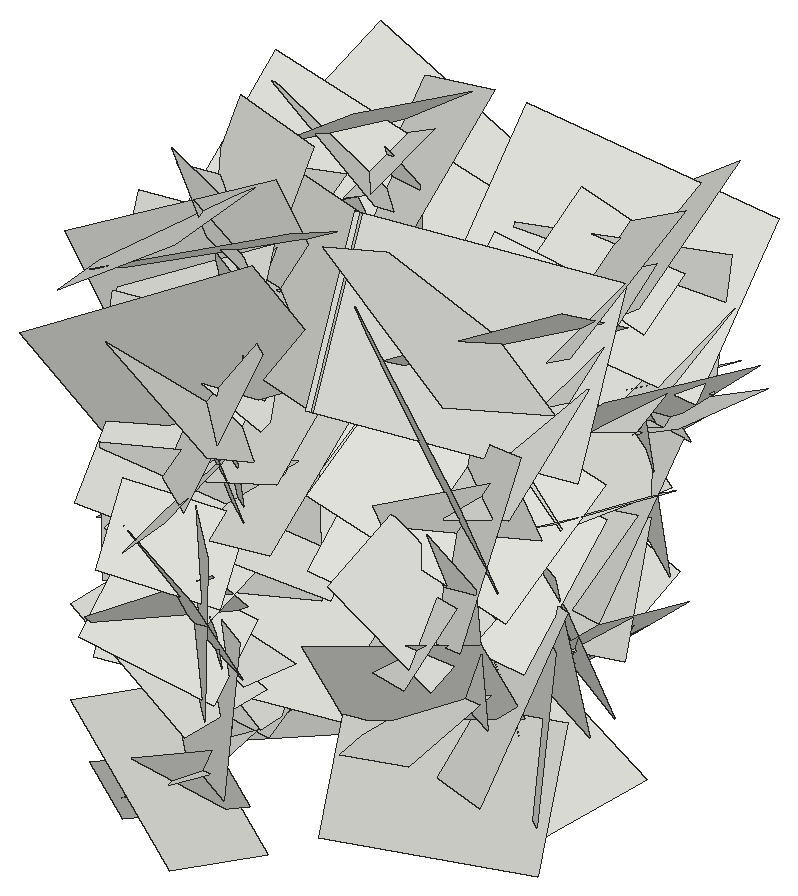
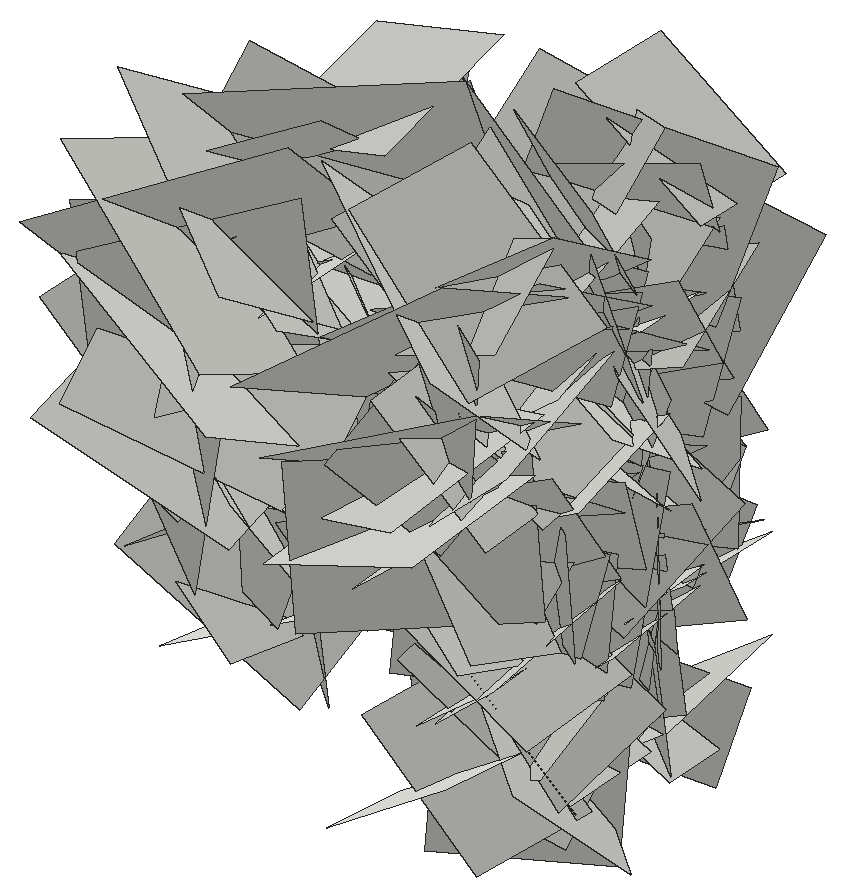
# SketchUp Ruby script. Lengths in inches.
U = 1.inch
M = Sketchup.active_model
def pt(a) = Geom::Point3d.new(a.map { |v| v * U })
def face(e, loops, mat)
  f = e.add_face(loops[0].map { |a| pt(a) })
  loops[1..].each { |l| e.add_face(l.map { |a| pt(a) }).erase! }
  f.material = f.back_material = mat if mat
  f
end
# faces: each face lists its corners as indices into pts; further lists are holes
def faces(e, pts, list, mat = nil) = list.each { |f| face(e, (f[0].is_a?(Array) ? f : [f]).map { |l| l.map { |i| pts[i] } }, mat) }
# xy, xz, yz: faces in a plane at the given z, y or x. An outline is a flat list of corners, or four numbers for a rectangle; further outlines are holes
def ring(l) = l.size == 4 ? [[l[0], l[1]], [l[2], l[1]], [l[2], l[3]], [l[0], l[3]]] : l.each_slice(2).to_a
def flat(e, list, mat, &to3) = list.each { |f| face(e, (f[0].is_a?(Array) ? f : [f]).map { |l| ring(l).map { |u, v| to3.(u, v) } }, mat) }
def xy(e, z, list, mat = nil) = flat(e, list, mat) { |x, y| [x, y, z] }
def xz(e, y, list, mat = nil) = flat(e, list, mat) { |x, z| [x, y, z] }
def yz(e, x, list, mat = nil) = flat(e, list, mat) { |y, z| [x, y, z] }
def lines(e, pts, list) = list.each { |a, b| e.add_line(pt(pts[a]), pt(pts[b])) }
# prism: a flat outline (further loops are holes) pulled along v
def prism(e, loops, v, mat = nil)
  f = face(e, loops, mat); d = Geom::Vector3d.new(v.map { |x| x * U })
  f.pushpull(f.normal.samedirection?(d) ? d.length : -d.length)
end
def box(e, o, s, mat = nil) = prism(e, [[o, [o[0] + s[0], o[1], o[2]], [o[0] + s[0], o[1] + s[1], o[2]], [o[0], o[1] + s[1], o[2]]]], [0, 0, s[2]], mat)
def at(x, y, z, deg = 0) = Geom::Transformation.translation(pt([x, y, z])) * Geom::Transformation.rotation(ORIGIN, Z_AXIS, deg.degrees)
def axes(o, x, y, z) = Geom::Transformation.new([*x, 0, *y, 0, *z, 0, *pt(o).to_a, 1])
def part(name) = M.definitions.add(name)
# library, detail: a bought-in or finely detailed component or shape, given as its bounding box
def library(name, o, s) = part(name).tap { |d| box(d.entities, o, s) }
def detail(e, o, s) = box(e.add_group.entities, o, s)
def put(e, d, t, mat = nil) = e.add_instance(d, t).tap { |i| i.material = mat if mat }
def group(e, t, mat = nil) = e.add_group.tap { |g| g.transformation = t; g.material = mat if mat }.entities
root = M.entities
c1 = part("Component\#6")
p = [[0.01,0,0],[0,3.24,4.54],[4.32,3.24,4.54],[4.33,0,0]]
faces(c1.entities,p,[[0,1,2,3]])
put(root,c1,axes([28.31,184.92,37.05],[-0.01613,-0.13323,-0.78421],[-0.01491,-0.78419,0.1335],[-0.84304,0.01642,0.01265]))
put(root,c1,axes([28.31,184.52,38.07],[0.06477,0.36641,0.7198],[-0.11209,0.71927,-0.35717],[-0.84878,-0.06703,0.10209]))
put(root,c1,axes([28.31,187.74,23.43],[0.08523,-0.9506,0.05636],[0.09187,0.06363,0.94959],[-1.00521,-0.07479,0.09156]))
put(root,c1,axes([24.34,187.08,35.11],[-0.23629,-0.52338,-1.02054],[-0.13084,-1.02265,0.55142],[1.20867,-0.21302,-0.13982]))
put(root,c1,axes([28.31,188.23,41.22],[0.26749,1.02168,-0.17372],[-0.00845,-0.17688,-1.05183],[-1.0985,0.25014,-0.03421]))
put(root,c1,axes([24.34,185.86,28.71],[-0.06844,0.29244,0.76285],[0.17475,0.75415,-0.27515],[0.84819,-0.13178,0.11824]))
put(root,c1,axes([24.34,192.58,32.17],[0.11188,-0.86522,-0.03173],[-0.14554,-0.04829,0.85998],[0.90613,0.09907,0.14204]))
put(root,c1,axes([24.34,189.53,40.3125],[-0.07096,0.70634,-0.4758],[0.12627,-0.46481,-0.70678],[0.89387,0.12173,0.06207]))
put(root,c1,axes([24.34,180.54,27.52],[0.00647,0.86334,-0.00303],[-0.00368,-0.003,-0.86336],[0.91514,-0.00612,-0.00345]))
put(root,c1,axes([28.31,184.84,39.1],[-0.02023,-0.20369,-0.6632],[-0.11732,-0.65406,0.20407],[-0.72599,0.11137,-0.0145]))
put(root,c1,axes([28.31,187.61,26.86],[0.07932,-0.16974,-0.83453],[0.0041,-0.83766,0.17072],[-0.9027,-0.01872,-0.07255]))
put(root,c1,axes([28.31,187.84,31.26],[-0.01205,0.8882,0.30464],[0.22592,0.29915,-0.86424],[-0.96935,0.05868,-0.20521]))
put(root,c1,axes([24.34,187.32,34.27],[0.05201,-0.4187,0.7383],[-0.02779,0.73844,0.42051],[0.89926,0.04704,-0.0297]))
put(root,c1,axes([28.31,182.78,23.92],[0.06221,-0.24398,0.83625],[0.07047,0.83695,0.23952],[-0.92069,0.04758,0.07484]))
put(root,c1,axes([24.34,186.99,20.26],[0.04681,-0.17583,0.86867],[-0.05724,0.86759,0.17835],[0.93771,0.06173,-0.03248]))
put(root,c1,axes([28.31,186.98,23.44],[0.07046,0.41434,0.63319],[-0.10971,0.63463,-0.40442],[-0.79457,-0.05088,0.11199]))
put(root,c1,axes([24.34,183.5625,38.07],[0.03427,-0.86867,-0.02883],[-0.01016,-0.0292,0.8692],[0.92124,0.03199,0.01066]))
put(root,c1,axes([24.34,189.58,22.99],[-0.08755,-0.94666,0.34405],[-0.04779,0.34833,0.94763],[1.06661,-0.0621,0.0707]))
put(root,c1,axes([28.31,194.3125,23.26],[0.02367,-0.75059,-0.08188],[-0.02978,-0.08269,0.75031],[-0.79979,-0.01914,-0.03036]))
put(root,c1,axes([24.34,191.48,24.4],[-0.24044,-0.84726,-0.84182],[-0.11443,-0.83882,0.87332],[1.26085,-0.2377,-0.08127]))
put(root,c1,axes([24.34,182.91,34.72],[-0.14912,-0.41506,0.98502],[-0.044,0.99488,0.41329],[1.13217,-0.016,0.1458]))
put(root,c1,axes([28.31,183.3,35.54],[-0.06853,-0.0517,0.64839],[-0.02911,0.65122,0.04919],[-0.68886,-0.02238,-0.06659]))
put(root,c1,axes([28.31,186.9,33.68],[0.12726,-0.80704,-0.07778],[-0.05104,-0.08559,0.81372],[-0.85791,-0.11462,-0.05995]))
put(root,c1,axes([24.34,189.24,21.76],[0.15995,-0.688,0.38857],[-0.02017,0.39231,0.70202],[0.83731,0.14088,-0.05731]))
put(root,c1,axes([24.34,190.89,25.45],[-0.07637,-0.93381,0.1535],[0.06656,0.14888,0.93522],[1.00091,-0.08115,-0.05048]))
put(root,c1,axes([28.31,181.75,22.9],[-0.07496,0.59984,0.04506],[-0.05269,0.03939,-0.60235],[-0.63545,-0.07402,0.04463]))
put(root,c1,axes([24.34,186.8,27.07],[-0.11611,-1.02809,0.5245],[-0.14127,0.5346,1.02006],[1.21522,-0.03608,0.16869]))
put(root,c1,axes([28.31,189.49,31],[0.19159,0.03614,-0.77666],[-0.1449,-0.78347,-0.06827],[-0.81131,0.14846,-0.17121]))
put(root,c1,axes([28.31,188.48,31.6],[-0.00806,0.51701,-0.38199],[-0.06142,-0.38101,-0.51453],[-0.67861,0.02834,0.0511]))
put(root,c1,axes([24.34,182.86,27.86],[0.00866,0.87216,-0.09866],[0.12421,-0.09886,-0.86427],[0.92206,0.00513,0.11735]))
put(root,c1,axes([28.31,188.3,31.13],[0.1103,-0.11339,-0.88165],[0.13763,-0.87621,0.12802],[-0.93214,-0.14279,-0.08543]))
put(root,c1,axes([24.34,182.62,33.52],[-0.16113,0.63843,0.91206],[-0.00988,0.91976,-0.64538],[1.18006,0.09488,0.11913]))
put(root,c1,axes([24.34,186.85,26],[0.04759,0.74401,-0.43208],[0.09551,-0.43435,-0.73856],[0.90698,0.0067,0.10045]))
put(root,c1,axes([28.31,188.01,25.87],[0.18323,0.88768,-0.1275],[0.06793,-0.14175,-0.89995],[-0.94816,0.16139,-0.08912]))
put(root,c1,axes([28.31,181.88,29.24],[-0.0732,0.47057,-0.46808],[0.06498,-0.46407,-0.47558],[-0.70054,-0.09222,0.00479]))
put(root,c1,axes([28.31,186.27,36.66],[0.23271,0.08267,-1.0169],[0.17131,-1.02986,-0.04883],[-1.06781,-0.14721,-0.22945]))
put(root,c1,axes([28.31,182.11,23.57],[0.01533,0.32032,-0.55846],[-0.07998,-0.55391,-0.31966],[-0.67773,0.07262,0.02509]))
put(root,c1,axes([24.34,181.12,36.49],[-0.0887,0.85058,-0.45713],[0.14057,-0.44437,-0.85112],[1.01388,0.13603,0.07801]))
put(root,c1,axes([24.34,184.8,33.37],[0.19651,0.19461,-0.78555],[-0.01158,-0.80522,-0.20206],[0.85778,-0.05545,0.17724]))
put(root,c1,axes([24.34,180.55,24.45],[0.04702,0.95483,-0.28451],[-0.08229,-0.28062,-0.95386],[1.05288,-0.06457,-0.06184]))
put(root,c1,axes([24.34,186.48,30.64],[0.03295,0.70699,0.47041],[0.18441,0.45544,-0.69599],[0.88105,-0.12176,0.12808]))
put(root,c1,axes([28.31,184.65,28.76],[-0.04824,-0.62434,-0.28052],[0.09786,-0.28417,0.61748],[-0.7189,0.00321,0.10288]))
put(root,c1,axes([28.31,188.62,32.29],[0.0866,-0.74743,0.19758],[0.06186,0.20408,0.74787],[-0.81715,-0.06376,0.07755]))
put(root,c1,axes([28.31,183.74,37.84],[-0.08456,-0.37494,0.46177],[0.03825,0.46199,0.38136],[-0.62935,0.07846,-0.03886]))
put(root,c1,axes([24.34,185.4,30.76],[-0.02152,-0.00963,-1.2106],[-0.23963,-1.18945,0.01326],[1.26071,-0.22625,-0.01814]))
put(root,c1,axes([24.34,187.18,35.87],[-0.21905,1.32848,-0.23139],[-0.18572,-0.25856,-1.32798],[1.41727,0.17144,-0.20979]))
put(root,c1,axes([28.31,188.41,35.3125],[-0.03073,0.48255,0.4704],[0.10717,0.46862,-0.47449],[-0.70624,0.05011,-0.09248]))
put(root,c1,axes([28.31,183.98,26.9],[0.15473,-0.64925,-0.29626],[-0.07231,-0.3137,0.65387],[-0.75301,-0.10329,-0.12366]))
put(root,c1,axes([28.31,183.4375,30.23],[0.10865,-0.24445,0.66529],[-0.00738,0.67183,0.24793],[-0.75127,-0.04195,0.09378]))
put(root,c1,axes([28.31,185.35,37.93],[0.06077,0.5182,0.40006],[-0.00909,0.40215,-0.51968],[-0.69387,0.04012,0.04185]))
put(root,c1,axes([24.34,182.41,31.86],[-0.21699,-0.67676,1.03332],[0.0082,1.04669,0.68705],[1.3093,-0.11872,0.16695]))
put(root,c1,axes([24.34,181.64,30.57],[0.02444,0.48831,-0.77146],[0.19424,-0.75848,-0.47462],[0.9481,0.1428,0.11713]))
put(root,c1,axes([24.34,184.85,32.98],[-0.15473,1.07562,-0.16592],[0.16403,-0.14519,-1.07739],[1.14193,0.1666,0.13228]))
put(root,c1,axes([28.31,179.78,31.84],[0.01485,0.68647,0.23212],[0.1576,0.2245,-0.67291],[-0.75179,0.06062,-0.13648]))
put(root,c1,axes([28.31,188.93,38.32],[0.06934,0.59373,0.25],[-0.00198,0.25145,-0.59671],[-0.68287,0.05956,0.02711]))
put(root,c1,axes([28.31,193.29,29.97],[-0.02765,-0.60791,0.13872],[0.08921,0.13414,0.60366],[-0.6549,0.04394,0.07638]))
put(root,c1,axes([24.34,189.07,22.99],[0.09993,-0.91741,-0.05408],[0.10319,-0.04408,0.91762],[0.96866,0.09934,-0.09218]))
put(root,c1,axes([24.34,185.63,37.94],[-0.10296,1.07287,0.66666],[-0.13207,0.65722,-1.07584],[1.33238,0.14805,-0.05512]))
put(root,c1,axes([24.34,185.55,26.35],[0.05433,-0.24183,-1.04679],[-0.06418,-1.04696,0.23891],[1.13701,-0.04754,0.0635]))
put(root,c1,axes([28.31,186.02,29.02],[0.12909,0.32312,-0.64935],[0.06195,-0.66067,-0.31779],[-0.76632,0.00102,-0.13508]))
put(root,c1,axes([24.34,190.19,31.82],[0.07854,-1.04848,0.11995],[-0.05802,0.11627,1.05008],[1.11713,0.07975,0.0461]))
put(root,c1,axes([28.31,188.83,29.07],[0.04972,0.59189,0.16701],[0.02122,0.16593,-0.59371],[-0.65156,0.05057,-0.00659]))
put(root,c1,axes([24.34,185.29,39.56],[0.11827,0.82487,-0.51088],[0.03346,-0.51706,-0.82795],[1.02793,-0.07808,0.08573]))
put(root,c1,axes([24.34,186.92,28.87],[0.11772,1.08189,-0.3436],[-0.18933,-0.32428,-1.0788],[1.18826,-0.15885,-0.13785]))
put(root,c1,axes([28.31,191.45,35.51],[0.13227,0.51495,-0.41011],[0.00116,-0.41758,-0.52399],[-0.6978,0.09692,-0.07861]))
put(root,c1,axes([28.31,183.51,30.36],[0.10644,-0.42009,-0.4575],[-0.01901,-0.46521,0.42323],[-0.65811,-0.0545,-0.08622]))
put(root,c1,axes([24.34,184.16,23.6],[0.00632,0.19994,1.20323],[-0.15077,1.19515,-0.1979],[1.28409,0.13934,-0.02916]))
put(root,c1,axes([24.34,189.26,31.29],[0.07003,-0.18149,-1.00879],[0.05402,-1.00905,0.18487],[1.08514,0.06195,0.0559]))
put(root,c1,axes([28.31,191.07,24.72],[0.08022,-0.60182,-0.03468],[0.03515,-0.03074,0.60586],[-0.63802,-0.07736,0.02902]))
put(root,c1,axes([24.34,187.65,25.55],[0.14301,-0.32766,0.90945],[0.11586,0.91755,0.31436],[1.01811,-0.05839,-0.16352]))
put(root,c1,axes([24.34,192.86,38.11],[0.10772,-0.0541,-1.0459],[0.04447,-1.04976,0.05837],[1.10925,0.04734,0.09923]))
put(root,c1,axes([28.31,188.74,27.6],[0.13014,-0.45431,-0.37588],[0.00674,-0.3829,0.46487],[-0.62498,-0.09873,-0.07326]))
put(root,c1,axes([24.34,181.98,27.65],[0.03848,-0.07343,1.06513],[0.13392,1.05855,0.06867],[1.12376,-0.12364,-0.04466]))
put(root,c1,axes([24.34,182.88,33.98],[0.05541,0.90127,0.55592],[0.17138,0.54328,-0.89597],[1.1093,-0.12895,0.11065]))
put(root,c1,axes([24.34,190.1,29],[0.15352,-0.05709,1.12322],[-0.06907,1.13017,0.06585],[1.19015,0.07295,-0.14107]))
put(root,c1,axes([24.34,185.59,36.56],[0.07365,1.00309,0.56692],[0.00038,0.56794,-1.00493],[1.22135,-0.06067,-0.03387]))
put(root,c1,axes([24.34,194.96,38.36],[-0.08597,-0.96025,-0.92678],[-0.03419,-0.92681,0.9631],[1.41421,-0.08078,-0.03305]))
put(root,c1,axes([24.34,188.57,34.3],[-0.02784,1.05016,0.5271],[0.1514,0.52617,-1.0412],[1.23628,-0.04079,0.13938]))
put(root,c1,axes([24.34,186.91,28.91],[-0.08475,0.77289,1.06783],[0.0494,1.07079,-0.77154],[1.39641,0.00903,0.0921]))
put(root,c1,axes([24.34,187.29,32.09],[-0.03087,-0.89426,-0.74249],[0.26998,-0.72958,0.86873],[1.20212,0.14089,-0.21417]))
put(root,c1,axes([24.34,190.5,33.59],[0.11278,1.05886,-0.21225],[0.21462,-0.22906,-1.04119],[1.12442,-0.06248,0.22002]))
put(root,c1,axes([24.34,184.99,36.41],[0.13687,-0.99381,0.45239],[0.15227,0.46704,0.985],[1.14738,0.05657,-0.18469]))
put(root,c1,axes([24.34,181.61,25.33],[-0.14764,0.72138,1.18272],[0.09804,1.19088,-0.71546],[1.46521,-0.007,0.16705]))
put(root,c1,axes([24.34,187.26,33.24],[0.066,-0.95024,-0.64083],[0.19237,-0.6255,0.94515],[1.19957,0.15259,-0.11631]))
put(root,c1,axes([24.34,188.72,38.18],[0.108,1.17484,0.54266],[-0.09899,0.5496,-1.17232],[1.36819,-0.05298,-0.12766]))
put(root,c1,axes([24.34,180.73,30.67],[0.05707,0.69485,1.12415],[-0.04583,1.1254,-0.69356],[1.4001,0.00851,-0.06852]))
put(root,c1,axes([24.34,188.1875,39.24],[0.00053,-0.50504,-1.25708],[0.1621,-1.24903,0.50186],[1.42684,0.14209,-0.05655]))
put(root,c1,axes([24.34,186.51,25.44],[-0.00901,-0.3677,1.34811],[0.26845,1.32541,0.3631],[1.45667,-0.24653,-0.05858]))
put(root,c1,axes([24.34,190.14,35.27],[0.30668,1.10496,-0.445],[0.14325,-0.48543,-1.11748],[1.25452,-0.21469,0.23639]))
put(root,c1,axes([38.11,190.14,35.27],[-0.30668,1.10496,-0.445],[-0.14325,-0.48543,-1.11748],[-1.25452,-0.21469,0.23639]))
put(root,c1,axes([38.11,186.51,25.44],[0.00901,-0.3677,1.34811],[-0.26845,1.32541,0.3631],[-1.45667,-0.24653,-0.05858]))
put(root,c1,axes([38.11,188.1875,39.24],[-0.00053,-0.50504,-1.25708],[-0.1621,-1.24903,0.50186],[-1.42684,0.14209,-0.05655]))
put(root,c1,axes([38.11,180.73,30.67],[-0.05707,0.69485,1.12415],[0.04583,1.1254,-0.69356],[-1.4001,0.00851,-0.06852]))
put(root,c1,axes([38.11,188.72,38.18],[-0.108,1.17484,0.54266],[0.09899,0.5496,-1.17232],[-1.36819,-0.05298,-0.12766]))
put(root,c1,axes([38.11,187.26,33.24],[-0.066,-0.95024,-0.64083],[-0.19237,-0.6255,0.94515],[-1.19957,0.15259,-0.11631]))
put(root,c1,axes([38.11,181.61,25.33],[0.14764,0.72138,1.18272],[-0.09804,1.19088,-0.71546],[-1.46521,-0.007,0.16705]))
put(root,c1,axes([38.11,184.99,36.41],[-0.13687,-0.99381,0.45239],[-0.15227,0.46704,0.985],[-1.14738,0.05657,-0.18469]))
put(root,c1,axes([38.11,190.5,33.59],[-0.11278,1.05886,-0.21225],[-0.21462,-0.22906,-1.04119],[-1.12442,-0.06248,0.22002]))
put(root,c1,axes([38.11,187.29,32.09],[0.03087,-0.89426,-0.74249],[-0.26998,-0.72958,0.86873],[-1.20212,0.14089,-0.21417]))
put(root,c1,axes([38.11,186.91,28.91],[0.08475,0.77289,1.06783],[-0.0494,1.07079,-0.77154],[-1.39641,0.00903,0.0921]))
put(root,c1,axes([38.11,188.57,34.3],[0.02784,1.05016,0.5271],[-0.1514,0.52617,-1.0412],[-1.23628,-0.04079,0.13938]))
put(root,c1,axes([38.11,194.96,38.36],[0.08597,-0.96025,-0.92678],[0.03419,-0.92681,0.9631],[-1.41421,-0.08078,-0.03305]))
put(root,c1,axes([38.11,185.59,36.56],[-0.07365,1.00309,0.56692],[-0.00038,0.56794,-1.00493],[-1.22135,-0.06067,-0.03387]))
put(root,c1,axes([38.11,190.1,29],[-0.15352,-0.05709,1.12322],[0.06907,1.13017,0.06585],[-1.19015,0.07295,-0.14107]))
put(root,c1,axes([38.11,182.88,33.98],[-0.05541,0.90127,0.55592],[-0.17138,0.54328,-0.89597],[-1.1093,-0.12895,0.11065]))
put(root,c1,axes([38.11,181.98,27.65],[-0.03848,-0.07343,1.06513],[-0.13392,1.05855,0.06867],[-1.12376,-0.12364,-0.04466]))
put(root,c1,axes([34.14,188.74,27.6],[-0.13014,-0.45431,-0.37588],[-0.00674,-0.3829,0.46487],[0.62498,-0.09873,-0.07326]))
put(root,c1,axes([38.11,192.86,38.11],[-0.10772,-0.0541,-1.0459],[-0.04447,-1.04976,0.05837],[-1.10925,0.04734,0.09923]))
put(root,c1,axes([38.11,187.65,25.55],[-0.14301,-0.32766,0.90945],[-0.11586,0.91755,0.31436],[-1.01811,-0.05839,-0.16352]))
put(root,c1,axes([34.14,191.07,24.72],[-0.08022,-0.60182,-0.03468],[-0.03515,-0.03074,0.60586],[0.63802,-0.07736,0.02902]))
put(root,c1,axes([38.11,189.26,31.29],[-0.07003,-0.18149,-1.00879],[-0.05402,-1.00905,0.18487],[-1.08514,0.06195,0.0559]))
put(root,c1,axes([38.11,184.16,23.6],[-0.00632,0.19994,1.20323],[0.15077,1.19515,-0.1979],[-1.28409,0.13934,-0.02916]))
put(root,c1,axes([34.14,183.51,30.36],[-0.10644,-0.42009,-0.4575],[0.01901,-0.46521,0.42323],[0.65811,-0.0545,-0.08622]))
put(root,c1,axes([34.14,191.45,35.51],[-0.13227,0.51495,-0.41011],[-0.00116,-0.41758,-0.52399],[0.6978,0.09692,-0.07861]))
put(root,c1,axes([38.11,186.92,28.87],[-0.11772,1.08189,-0.3436],[0.18933,-0.32428,-1.0788],[-1.18826,-0.15885,-0.13785]))
put(root,c1,axes([38.11,185.29,39.56],[-0.11827,0.82487,-0.51088],[-0.03346,-0.51706,-0.82795],[-1.02793,-0.07808,0.08573]))
put(root,c1,axes([34.14,188.83,29.07],[-0.04972,0.59189,0.16701],[-0.02122,0.16593,-0.59371],[0.65156,0.05057,-0.00659]))
put(root,c1,axes([38.11,190.19,31.82],[-0.07854,-1.04848,0.11995],[0.05802,0.11627,1.05008],[-1.11713,0.07975,0.0461]))
put(root,c1,axes([34.14,186.02,29.02],[-0.12909,0.32312,-0.64935],[-0.06195,-0.66067,-0.31779],[0.76632,0.00102,-0.13508]))
put(root,c1,axes([38.11,185.55,26.35],[-0.05433,-0.24183,-1.04679],[0.06418,-1.04696,0.23891],[-1.13701,-0.04754,0.0635]))
put(root,c1,axes([38.11,185.63,37.94],[0.10296,1.07287,0.66666],[0.13207,0.65722,-1.07584],[-1.33238,0.14805,-0.05512]))
put(root,c1,axes([38.11,189.07,22.99],[-0.09993,-0.91741,-0.05408],[-0.10319,-0.04408,0.91762],[-0.96866,0.09934,-0.09218]))
put(root,c1,axes([34.14,193.29,29.97],[0.02765,-0.60791,0.13872],[-0.08921,0.13414,0.60366],[0.6549,0.04394,0.07638]))
put(root,c1,axes([34.14,188.93,38.32],[-0.06934,0.59373,0.25],[0.00198,0.25145,-0.59671],[0.68287,0.05956,0.02711]))
put(root,c1,axes([34.14,179.78,31.84],[-0.01485,0.68647,0.23212],[-0.1576,0.2245,-0.67291],[0.75179,0.06062,-0.13648]))
put(root,c1,axes([38.11,184.85,32.98],[0.15473,1.07562,-0.16592],[-0.16403,-0.14519,-1.07739],[-1.14193,0.1666,0.13228]))
put(root,c1,axes([38.11,181.64,30.57],[-0.02444,0.48831,-0.77146],[-0.19424,-0.75848,-0.47462],[-0.9481,0.1428,0.11713]))
put(root,c1,axes([38.11,182.41,31.86],[0.21699,-0.67676,1.03332],[-0.0082,1.04669,0.68705],[-1.3093,-0.11872,0.16695]))
put(root,c1,axes([34.14,185.35,37.93],[-0.06077,0.5182,0.40006],[0.00909,0.40215,-0.51968],[0.69387,0.04012,0.04185]))
put(root,c1,axes([34.14,183.4375,30.23],[-0.10865,-0.24445,0.66529],[0.00738,0.67183,0.24793],[0.75127,-0.04195,0.09378]))
put(root,c1,axes([34.14,183.98,26.9],[-0.15473,-0.64925,-0.29626],[0.07231,-0.3137,0.65387],[0.75301,-0.10329,-0.12366]))
put(root,c1,axes([34.14,188.41,35.3125],[0.03073,0.48255,0.4704],[-0.10717,0.46862,-0.47449],[0.70624,0.05011,-0.09248]))
put(root,c1,axes([38.11,187.18,35.87],[0.21905,1.32848,-0.23139],[0.18572,-0.25856,-1.32798],[-1.41727,0.17144,-0.20979]))
